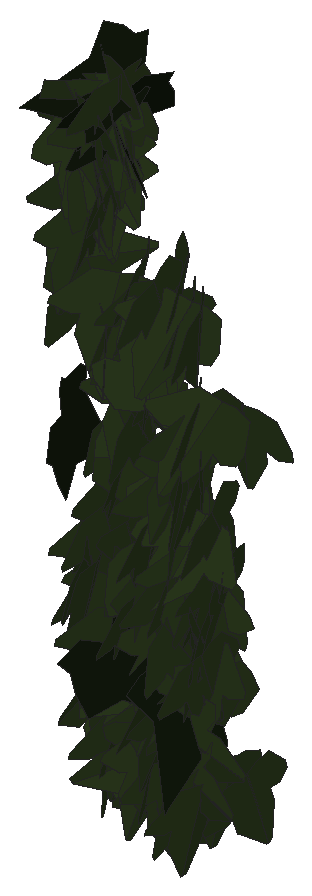
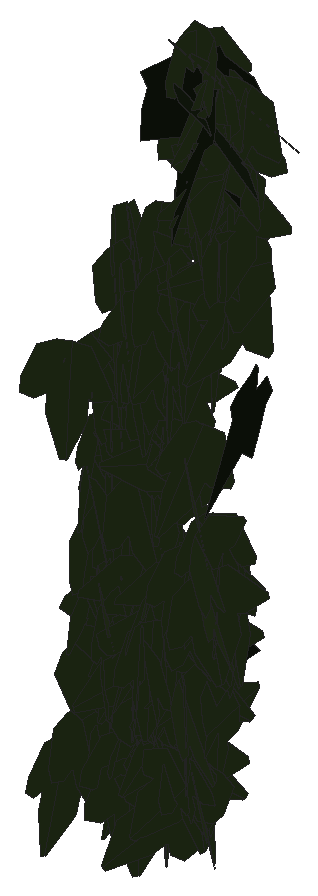
# SketchUp Ruby script. Lengths in inches.
U = 1.inch
M = Sketchup.active_model
def pt(a) = Geom::Point3d.new(a.map { |v| v * U })
def face(e, loops, mat)
  f = e.add_face(loops[0].map { |a| pt(a) })
  loops[1..].each { |l| e.add_face(l.map { |a| pt(a) }).erase! }
  f.material = f.back_material = mat if mat
  f
end
# faces: each face lists its corners as indices into pts; further lists are holes
def faces(e, pts, list, mat = nil) = list.each { |f| face(e, (f[0].is_a?(Array) ? f : [f]).map { |l| l.map { |i| pts[i] } }, mat) }
# xy, xz, yz: faces in a plane at the given z, y or x. An outline is a flat list of corners, or four numbers for a rectangle; further outlines are holes
def ring(l) = l.size == 4 ? [[l[0], l[1]], [l[2], l[1]], [l[2], l[3]], [l[0], l[3]]] : l.each_slice(2).to_a
def flat(e, list, mat, &to3) = list.each { |f| face(e, (f[0].is_a?(Array) ? f : [f]).map { |l| ring(l).map { |u, v| to3.(u, v) } }, mat) }
def xy(e, z, list, mat = nil) = flat(e, list, mat) { |x, y| [x, y, z] }
def xz(e, y, list, mat = nil) = flat(e, list, mat) { |x, z| [x, y, z] }
def yz(e, x, list, mat = nil) = flat(e, list, mat) { |y, z| [x, y, z] }
def lines(e, pts, list) = list.each { |a, b| e.add_line(pt(pts[a]), pt(pts[b])) }
# prism: a flat outline (further loops are holes) pulled along v
def prism(e, loops, v, mat = nil)
  f = face(e, loops, mat); d = Geom::Vector3d.new(v.map { |x| x * U })
  f.pushpull(f.normal.samedirection?(d) ? d.length : -d.length)
end
def box(e, o, s, mat = nil) = prism(e, [[o, [o[0] + s[0], o[1], o[2]], [o[0] + s[0], o[1] + s[1], o[2]], [o[0], o[1] + s[1], o[2]]]], [0, 0, s[2]], mat)
def at(x, y, z, deg = 0) = Geom::Transformation.translation(pt([x, y, z])) * Geom::Transformation.rotation(ORIGIN, Z_AXIS, deg.degrees)
def axes(o, x, y, z) = Geom::Transformation.new([*x, 0, *y, 0, *z, 0, *pt(o).to_a, 1])
def part(name) = M.definitions.add(name)
# library, detail: a bought-in or finely detailed component or shape, given as its bounding box
def library(name, o, s) = part(name).tap { |d| box(d.entities, o, s) }
def detail(e, o, s) = box(e.add_group.entities, o, s)
def put(e, d, t, mat = nil) = e.add_instance(d, t).tap { |i| i.material = mat if mat }
def group(e, t, mat = nil) = e.add_group.tap { |g| g.transformation = t; g.material = mat if mat }.entities
root = M.entities
M.materials.add("efeu1").color = [18, 25, 13]
M.materials.add("efeu2").color = [43, 57, 29]
c1 = part("ivyleaf_10")
p = [[0,0.5,-0.03],[-0.0625,2.02,-0.43],[-0.19,2.01,-0.46],[-0.54,1.05,-0.29],[-0.52,0.625,-0.18],[-0.83,0.76,-0.28],
  [-1.16,0.64,-0.33],[-1.15,0.33,-0.24],[-0.77,-0.39,0.02],[-0.3,-0.51,0.16],[0.04,-0.48,0.23],[-0.02,2.01,-0.4375],
  [-0.06,2.01,-0.43],[0.04,-0.49,0.23],[0.67,-0.49,0.14],[1.38,0.36,-0.2],[1.375,0.51,-0.24],[0.81,0.65,-0.19],
  [0.62,0.59,-0.15],[0.6,1.09,-0.28],[0.5,1.23,-0.31]]
faces(c1.entities,p,[[0,1,2,3,4,5,6,7,8,9,10],[11,12,0,13,14,15,16,17,18,19,20]],"efeu2")
c2 = part("ivyleaf_9")
p = [[1.54,2.16,1.25],[1.36,2.04,1.19],[-0.21,0.99,0.68],[-0.71,1.11,0.82],[-0.85,0.86,0.67],[-0.8,0.17,0.21],
  [-0.9,-0.01,0.1],[-0.67,-0.16,-0.02],[-0.08,-0.08,-0.05],[-0.03,-0.6,-0.4],[0.65,-0.88,-0.66],[0.83,-0.6,-0.49],
  [1.29,-0.42,-0.43],[1.8125,-0.07,-0.26],[1.21,0.44,0.15]]
faces(c2.entities,p,[[0,1,2,3,4,5,6,7,8,9,10,11,12,13,14]],"efeu1")
put(root,c1,axes([11.7,225.35,216.89],[-0.17857,-0.46173,0.07016],[0.01212,-0.07967,-0.49346],[0.46687,-0.17454,0.03964]))
put(root,c1,axes([11.74,225.21,216.97],[0.16413,-0.47089,0.03635],[0.00143,-0.03798,-0.49855],[0.47229,0.16376,-0.01112]))
put(root,c1,axes([11.82,224.86,221.38],[-0.39838,-0.30173,0.01575],[-0.01265,-0.00938,-0.49975],[0.30188,-0.39858,-0.00016]))
put(root,c1,axes([11.73,225.29,217.39],[0.11032,-0.44113,0.20794],[0.06177,-0.19884,-0.45459],[0.48375,0.12599,0.01063]))
put(root,c1,axes([11.78,224.85,220.93],[-0.07095,-0.43919,0.2282],[0.07533,-0.23743,-0.43353],[0.48917,-0.02713,0.09986]))
put(root,c1,axes([11.84,225.46,215.62],[0.11046,-0.48106,0.07989],[0.00859,-0.07998,-0.49349],[0.48757,0.11039,-0.0094]))
put(root,c2,axes([11.9,224.29,218.81],[0.12477,-0.03223,-0.48311],[-0.37094,0.31428,-0.11676],[0.31119,0.38754,0.05452]))
put(root,c1,axes([11.77,224.71,220.16],[-0.14135,-0.32481,-0.35287],[0.14656,0.32103,-0.3542],[0.45667,-0.20356,0.00445]))
put(root,c1,axes([11.9,224.64,216.87],[0.05893,-0.33516,-0.36632],[-0.04723,0.36344,-0.34012],[0.49426,0.07469,0.01118]))
put(root,c1,axes([11.87,224.78,216.61],[0.0968,-0.48951,-0.03181],[-0.00242,0.03195,-0.49897],[0.49054,0.09675,0.00381]))
put(root,c1,axes([11.77,224.7,222.57],[-0.4744,-0.04279,-0.15202],[0.15347,-0.01139,-0.47573],[0.03725,-0.49804,0.02394]))
put(root,c1,axes([11.86,225.47,215.66],[0.23212,-0.41432,-0.15639],[-0.00102,0.17606,-0.46798],[0.44285,0.21758,0.08089]))
put(root,c1,axes([11.8125,225.09,215.1875],[-0.04659,0.03065,-0.49688],[-0.01642,-0.49887,-0.02923],[-0.49755,0.0136,0.04749]))
put(root,c1,axes([11.86,224.875,221.74],[-0.28903,0.40568,-0.04344],[-0.00216,-0.05475,-0.49699],[-0.40799,-0.2871,0.0334]))
put(root,c2,axes([12.22,224.72,222.37],[-0.19027,0.37137,0.27547],[-0.20623,0.19845,-0.40999],[-0.41385,-0.26963,0.07765]))
put(root,c1,axes([11.96,225.22,216.58],[-0.10841,-0.45411,0.17896],[-0.0212,-0.17877,-0.46647],[0.48765,-0.10872,0.01951]))
put(root,c1,axes([11.82,224.77,221.83],[-0.4552,0.11573,-0.17145],[0.1371,-0.14153,-0.45953],[-0.1549,-0.46538,0.09712]))
put(root,c1,axes([11.6875,224.625,220.59],[-0.0317,-0.04118,-0.49729],[0.34536,0.35785,-0.05165],[0.36017,-0.34676,0.00576]))
put(root,c1,axes([11.89,224.71,222.08],[0.47557,0.14781,-0.04451],[-0.06545,0.06248,-0.49175],[-0.13981,0.47355,0.07877]))
put(root,c1,axes([11.86,224.86,221.53],[0.02828,0.49288,0.07916],[-0.00436,0.07953,-0.49362],[-0.49918,0.02723,0.00879]))
put(root,c1,axes([11.89,225.22,214.49],[0.26255,-0.42121,0.06046],[0.06203,-0.03241,-0.49508],[0.42098,0.26746,0.03523]))
put(root,c1,axes([11.99,224.7,221.3],[0.18623,-0.38989,-0.25159],[-0.0422,0.25575,-0.42757],[0.4621,0.18049,0.06235]))
put(root,c1,axes([11.87,224.92,221.62],[0.14253,0.47795,0.0353],[0.0153,0.03228,-0.49872],[-0.47901,0.14324,-0.00543]))
put(root,c2,axes([12.31,224.76,222.93],[-0.41203,0.23888,0.15221],[-0.16527,0.01546,-0.47164],[-0.23004,-0.43897,0.06622]))
put(root,c1,axes([11.99,224.57,222.52],[-0.41687,0.27608,0.00038],[0.00032,0.00117,-0.5],[-0.27608,-0.41687,-0.00115]))
put(root,c1,axes([11.99,224.9,217.32],[-0.06332,-0.46543,-0.17136],[0.07804,0.16125,-0.46681],[0.4898,-0.08586,0.05223]))
put(root,c1,axes([12.05,225.15,214.67],[-0.09041,-0.491,0.02737],[0.01637,-0.03082,-0.49878],[0.49149,-0.0893,0.02165]))
put(root,c1,axes([11.78,224.93,221.86],[0.36756,0.20326,0.27127],[0.21144,0.17526,-0.41782],[-0.26493,0.42187,0.04288]))
put(root,c1,axes([12.06,225.21,217.03],[-0.1396,-0.44702,-0.17517],[0.04992,0.16792,-0.46831],[0.47751,-0.14824,-0.00225]))
put(root,c1,axes([12.14,224.92,216.05],[-0.18571,-0.45465,0.09381],[-0.01438,-0.09535,-0.49061],[0.46401,-0.18492,0.02234]))
put(root,c1,axes([12.03,225.1,218.49],[-0.07518,-0.40489,-0.28357],[0.12073,0.2631,-0.40768],[0.47935,-0.12977,0.05821]))
put(root,c1,axes([12.15,224.63,219.82],[0.27561,-0.2664,-0.32105],[-0.10337,0.32917,-0.36189],[0.40417,0.26585,0.12637]))
put(root,c1,axes([12.11,224.96,221.53],[0.14162,-0.46694,-0.10911],[-0.01395,0.10971,-0.48761],[0.47932,0.14116,0.01805]))
put(root,c1,axes([12.11,225.05,218.07],[0.24396,-0.43277,-0.05648],[-0.01288,0.05754,-0.49651],[0.43625,0.24371,0.01692]))
put(root,c2,axes([12.19,224.82,222.4],[0.28676,0.01346,-0.40937],[-0.39923,0.12087,-0.27569],[0.09154,0.48498,0.08007]))
put(root,c1,axes([11.86,225.34,214.63],[0.26831,0.24909,0.34054],[0.21725,0.26439,-0.36456],[-0.36168,0.34359,0.03364]))
put(root,c1,axes([12.42,224.94,216.54],[-0.32834,0.02811,0.37603],[-0.37511,0.02655,-0.32953],[-0.03849,-0.4985,0.00366]))
put(root,c1,axes([12.17,224.79,222.375],[-0.27662,-0.41372,0.04816],[0.02211,-0.07232,-0.49425],[0.41592,-0.27131,0.0583]))
put(root,c1,axes([12.17,225,219.88],[0.06136,-0.46995,-0.15931],[0.0263,0.16338,-0.47182],[0.49552,0.04952,0.04477]))
put(root,c2,axes([12.31,224.77,222.75],[-0.01911,0.42881,-0.25644],[-0.0113,-0.25693,-0.42879],[-0.49951,-0.01059,0.01951]))
put(root,c1,axes([12.33,225.1,215.57],[0.25511,0.18186,-0.38967],[-0.31292,-0.23227,-0.31326],[-0.29496,0.40371,-0.0047]))
put(root,c1,axes([12.12,224.8,222.38],[-0.11924,0.48341,-0.04581],[0.00443,-0.04608,-0.49785],[-0.48555,-0.11913,0.00671]))
put(root,c1,axes([12.23,225.22,215.54],[-0.15709,-0.45485,0.13578],[0.01622,-0.14808,-0.47729],[0.4744,-0.14556,0.06128]))
put(root,c1,axes([12.23,224.77,220.27],[-0.31528,-0.36096,0.1425],[0.01916,-0.19785,-0.45879],[0.3876,-0.28384,0.13858]))
put(root,c1,axes([12.11,225.44,214.81],[0.48585,-0.11243,0.03617],[0.03624,-0.00384,-0.49867],[0.11241,0.48718,0.00442]))
put(root,c1,axes([12.1,224.73,222.6875],[-0.44305,0.10276,-0.20772],[0.142,-0.2338,-0.41854],[-0.18315,-0.42986,0.17798]))
put(root,c1,axes([12.24,224.79,222.56],[-0.24143,0.43682,0.02996],[-0.02765,0.01894,-0.49888],[-0.43698,-0.24254,0.01502]))
put(root,c1,axes([12.24,224.72,223.02],[-0.39495,0.29622,-0.07919],[0.04186,-0.07584,-0.49244],[-0.30375,-0.3956,0.0351]))
put(root,c1,axes([12.18,225.25,215.24],[-0.11074,-0.35966,-0.32921],[0.19214,0.27809,-0.36844],[0.44813,-0.20812,0.07662]))
put(root,c1,axes([12.3,225.1,220.42],[0.19276,-0.45725,-0.0614],[-0.00466,0.06461,-0.49579],[0.46133,0.1917,0.02065]))
put(root,c1,axes([12.31,225.48,216.15],[-0.12834,-0.47237,-0.10196],[0.03531,0.09604,-0.48942],[0.48196,-0.13283,0.00871]))
put(root,c1,axes([12.61,225.01,214.54],[0.20201,0.11662,-0.44226],[-0.43612,-0.09656,-0.22467],[-0.13782,0.47652,0.06271]))
put(root,c1,axes([12.1,225.36,214.17],[0.23558,0.20855,0.3886],[0.21214,0.33266,-0.30714],[-0.38665,0.30958,0.06825]))
put(root,c1,axes([12.46,225.05,219.03],[-0.33195,-0.31877,0.19544],[-0.06624,-0.20708,-0.45026],[0.368,-0.32482,0.09524]))
put(root,c1,axes([12.39,224.59,222.93],[-0.07749,-0.48516,-0.09283],[0.02034,0.09075,-0.49127],[0.49354,-0.07991,0.00567]))
put(root,c1,axes([12.43,224.8125,216.42],[0.09581,-0.47999,-0.10213],[-0.01398,0.10135,-0.48942],[0.49053,0.09664,0.006]))
put(root,c1,axes([12.35,225.55,216.02],[0.40714,-0.29006,0.01],[0.05538,0.06073,-0.4932],[0.2849,0.40271,0.08158]))
put(root,c1,axes([12.5,225.07,215.21],[0.08449,-0.4612,-0.17366],[-0.05038,0.16719,-0.46852],[0.49023,0.09667,-0.01822]))
put(root,c1,axes([12.5,225.07,220.21],[-0.09235,-0.48704,0.06531],[-0.00074,-0.06632,-0.49558],[0.4914,-0.09163,0.01153]))
put(root,c1,axes([12.36,225.04,216.8],[0.13746,0.47717,0.05843],[0.01659,0.05603,-0.49657],[-0.48045,0.13846,-0.00043]))
put(root,c1,axes([12.49,225.09,214.41],[0.24604,-0.39771,-0.17688],[-0.03368,0.18518,-0.46322],[0.43397,0.23986,0.06433]))
put(root,c1,axes([12.6875,225.33,215.45],[-0.20477,-0.19889,0.4105],[-0.22418,-0.348,-0.28043],[0.39726,-0.2989,0.05334]))
put(root,c1,axes([12.47,225.21,214.46],[-0.11519,-0.42075,0.24434],[0.07751,-0.26376,-0.41764],[0.48034,-0.05834,0.12598]))
put(root,c1,axes([12.5,225.48,216.1],[0.26301,-0.35921,-0.22758],[-0.02287,0.25526,-0.42932],[0.42462,0.23624,0.11784]))
put(root,c1,axes([12.53,225.01,219.46],[-0.1429,-0.46934,0.09646],[0.02579,-0.10804,-0.48751],[0.47845,-0.13435,0.05509]))
put(root,c1,axes([12.18,224.9,218.18],[-0.04808,-0.01631,-0.49742],[0.44719,0.21791,-0.05037],[0.21843,-0.44972,-0.00637]))
put(root,c1,axes([12.55,224.9,219.4],[0.2943,-0.34399,-0.21228],[-0.03936,0.23694,-0.43853],[0.40229,0.27482,0.11239]))
put(root,c2,axes([12.3125,224.63,215.95],[-0.03133,-0.11281,-0.4861],[0.16898,0.45588,-0.11669],[0.46953,-0.1716,0.00956]))
put(root,c1,axes([12.55,225.3,216.3],[0.11156,-0.40822,-0.2663],[0.0924,0.28594,-0.39962],[0.47856,0.03995,0.13924]))
put(root,c1,axes([12.66,225.26,217.74],[-0.17964,-0.4569,0.09471],[-0.0148,-0.09585,-0.4905],[0.46638,-0.17903,0.02091]))
put(root,c1,axes([12.62,224.59,218.9],[0.06869,-0.38267,-0.3144],[0.01754,0.31909,-0.38454],[0.49495,0.04179,0.05726]))
put(root,c1,axes([12.46,225.26,215.8],[0.10388,0.0892,0.48089],[0.08852,0.48007,-0.10817],[-0.48101,0.10761,0.08394]))
put(root,c1,axes([12.61,225.15,219.93],[-0.23462,-0.39609,-0.1951],[0.08756,0.17481,-0.46019],[0.43276,-0.25011,-0.01267]))
put(root,c1,axes([12.6,225.25,216.04],[0.04804,0.39124,0.30761],[-0.02582,0.31058,-0.39099],[-0.49702,0.02168,0.05005]))
put(root,c1,axes([12.71,224.78,217.5],[0.11997,-0.47747,-0.08734],[-0.00617,0.08846,-0.49207],[0.48536,0.11914,0.01533]))
put(root,c1,axes([12.8125,225.11,216.01],[-0.23104,-0.38865,0.21348],[-0.07507,-0.20296,-0.45075],[0.43702,-0.24033,0.03543]))
put(root,c1,axes([12.43,224.79,219.64],[0.37974,0.12884,0.29867],[0.27433,0.11982,-0.40048],[-0.17477,0.46802,0.02031]))
put(root,c1,axes([12.76,225.11,219.32],[0.04343,-0.48297,-0.12186],[-0.01123,0.12135,-0.48492],[0.49798,0.04486,-0.00031]))
put(root,c1,axes([12.75,224.64,219.37],[0.18629,0.46399,-0.00285],[0.00103,0.00265,0.49999],[0.464,-0.1863,0.00003]))
put(root,c1,axes([12.82,225.11,214.14],[-0.36164,-0.34518,0.00857],[-0.00542,-0.00673,-0.49993],[0.34524,-0.36167,0.00113]))
put(root,c1,axes([12.67,225.26,216.84],[0.15426,0.46817,0.08381],[0.00074,0.08788,-0.49222],[-0.47561,0.15198,0.02642]))
put(root,c1,axes([12.79,224.94,216.73],[-0.32618,-0.37176,-0.07348],[0.05142,0.05263,-0.49456],[0.37545,-0.33018,0.0039]))
put(root,c1,axes([12.69,225.08,216.41],[-0.12521,-0.32839,-0.35565],[0.1867,0.30617,-0.34843],[0.44662,-0.22005,0.04595]))
put(root,c1,axes([12.86,225.46,216.23],[0.03439,-0.46726,-0.17459],[0.00122,0.17509,-0.46834],[0.49881,0.03178,0.01318]))
put(root,c1,axes([12.5625,225.16,218.15],[0.38723,0.12393,0.29103],[0.25496,0.15,-0.40311],[-0.18723,0.46059,0.05297]))
put(root,c1,axes([12.72,225.16,214.7],[0.27436,-0.31209,0.27807],[0.20825,-0.18634,-0.41462],[0.36243,0.34333,0.02774]))
put(root,c1,axes([13.21,225.47,215.65],[-0.25754,-0.07725,0.42155],[-0.37396,-0.19973,-0.26507],[0.20935,-0.45182,0.0451]))
put(root,c1,axes([12.92,224.89,215.27],[0.06105,-0.47705,0.13673],[0.00065,-0.13769,-0.48067],[0.49626,0.05887,-0.0162]))
put(root,c1,axes([12.9,224.99,216.68],[-0.39379,0.30799,0.00859],[-0.00486,0.00772,-0.49992],[-0.30807,-0.39381,-0.00309]))
put(root,c1,axes([12.93,225.04,214.42],[-0.30919,-0.38377,-0.08438],[0.05719,0.06228,-0.4928],[0.38875,-0.31439,0.00538]))
put(root,c1,axes([12.95,225.12,220.125],[0.19475,-0.45122,-0.09205],[0.00887,0.1036,-0.48907],[0.46043,0.18886,0.04836]))
put(root,c1,axes([12.95,224.55,220.62],[-0.01572,-0.44709,-0.22331],[0.04534,0.22122,-0.4461],[0.49769,-0.03427,0.03359]))
put(root,c1,axes([13.01,225.39,216.55],[0.20504,-0.44577,-0.09619],[-0.04263,0.08627,-0.49065],[0.45403,0.2094,-0.00263]))
put(root,c1,axes([13,224.95,220.75],[0.25821,-0.40021,-0.1522],[-0.03706,0.15618,-0.47353],[0.42656,0.25582,0.05099]))
put(root,c1,axes([12.9,225.36,216.38],[-0.47488,-0.06954,-0.14018],[0.1522,-0.1012,-0.4654],[0.03635,-0.48469,0.11728]))
put(root,c1,axes([13.01,224.89,216.9375],[0.10308,-0.45738,-0.17372],[0.00338,0.17819,-0.46716],[0.48925,0.09513,0.03983]))
put(root,c1,axes([13.14,224.79,220.25],[-0.33323,-0.2728,0.25404],[-0.08132,-0.27934,-0.40664],[0.36379,-0.31233,0.1418]))
put(root,c1,axes([13.05,225.1,215.9],[0.23674,-0.37435,-0.23198],[-0.0029,0.26205,-0.42582],[0.44039,0.20296,0.12191]))
put(root,c1,axes([13.11,224.95,218.45],[-0.07865,-0.41668,0.26493],[0.03957,-0.27273,-0.4172],[0.49219,-0.04465,0.07588]))
put(root,c1,axes([13.05,224.6875,216.35],[0.04961,-0.40421,-0.29009],[0.11297,0.29307,-0.38903],[0.48454,-0.02694,0.12041]))
put(root,c1,axes([13.13,224.71,216.91],[-0.2141,-0.43776,-0.11193],[0.03741,0.10627,-0.48714],[0.45029,-0.21697,-0.01275]))
put(root,c1,axes([13.28,225.04,215.54],[-0.15612,-0.29742,0.37036],[-0.15294,-0.33761,-0.3356],[0.44971,-0.21807,0.01444]))
put(root,c1,axes([13.14,224.77,214.32],[0.0437,-0.41534,-0.27492],[0.07771,0.27828,-0.40807],[0.49199,-0.00706,0.08888]))
put(root,c1,axes([13.21,224.92,218.78],[-0.05356,-0.4646,0.17687],[0.00656,-0.17854,-0.46699],[0.49708,-0.0477,0.02522]))
put(root,c1,axes([13.26,224.55,218.38],[0.21495,-0.31404,-0.32431],[-0.08792,0.32319,-0.37124],[0.4428,0.21662,0.08372]))
put(root,c2,axes([13.05,225,215.43],[-0.02338,-0.47419,0.15684],[-0.01056,-0.15651,-0.47476],[0.49934,-0.02552,-0.0027]))
put(root,c1,axes([13.26,224.91,217.17],[-0.1694,-0.44472,0.15338],[0.00833,-0.16583,-0.47162],[0.47036,-0.15723,0.06359]))
put(root,c1,axes([13.25,224.85,219.06],[0.17785,-0.43292,-0.17592],[-0.0286,0.17779,-0.46645],[0.46642,0.17598,0.03848]))
put(root,c1,axes([13.05,224.92,218.02],[0.20632,-0.30168,0.3412],[0.23416,-0.25102,-0.36354],[0.39064,0.3098,0.0377]))
put(root,c1,axes([13.3,224.77,217.64],[0.45071,0.10303,-0.19037],[-0.18331,-0.05218,-0.46225],[-0.11512,0.48648,-0.00926]))
put(root,c1,axes([13.27,225.04,216.41],[0.20764,-0.41617,-0.18355],[-0.00611,0.1992,-0.45857],[0.4548,0.19268,0.07764]))
put(root,c1,axes([13.34,224.78,218.25],[0.13561,-0.38687,-0.28625],[-0.0597,0.28158,-0.40884],[0.47754,0.14506,0.03018]))
put(root,c1,axes([13.33,225.25,216.95],[0.02481,-0.49937,-0.00388],[-0.0022,0.00377,-0.49998],[0.49938,0.02482,-0.00201]))
put(root,c1,axes([13.3,225.19,217.47],[0.37445,-0.31863,-0.09087],[-0.03518,0.09812,-0.48902],[0.32946,0.37262,0.05106]))
put(root,c1,axes([13.23,225.48,216.5],[-0.04418,0.29484,-0.4014],[0.00759,-0.40253,-0.2965],[-0.49799,-0.03229,0.03109]))
put(root,c1,axes([13.45,224.9,219.07],[-0.31462,-0.26426,0.28492],[-0.0984,-0.30047,-0.38734],[0.37594,-0.29981,0.13706]))
put(root,c1,axes([13.22,225.0625,215.91],[0.49206,-0.0398,0.0793],[0.07856,-0.01225,-0.49364],[0.04123,0.49826,-0.0058]))
put(root,c1,axes([13.39,224.75,214.37],[-0.04985,-0.49653,0.03124],[0.0044,-0.03183,-0.49897],[0.49749,-0.04947,0.00754]))
put(root,c1,axes([13.43,224.79,216.03],[-0.08197,-0.45124,-0.19915],[0.04995,0.19325,-0.45843],[0.4907,-0.09505,0.0134]))
put(root,c1,axes([13.48,225.17,214.57],[-0.14419,-0.4756,0.05491],[-0.00759,-0.05506,-0.4969],[0.4787,-0.14413,0.00866]))
put(root,c1,axes([13.11,224.87,214.6],[-0.07142,0.0321,-0.49383],[0.40953,-0.27627,-0.07719],[-0.27782,-0.4155,0.01317]))
put(root,c1,axes([13.49,224.59,220.4],[0.17067,-0.44584,-0.14866],[0.00312,0.15923,-0.47396],[0.46996,0.16085,0.05714]))
put(root,c1,axes([13.11,224.91,215.02],[-0.05911,0.04153,-0.49475],[0.44254,-0.22148,-0.07146],[-0.22509,-0.44634,-0.01057]))
put(root,c1,axes([13.54,225.45,214.3],[-0.09237,-0.45298,-0.19046],[0.06626,0.18054,-0.46153],[0.48691,-0.1105,0.02667]))
put(root,c1,axes([13.58,224.78,217.92],[0.01475,-0.4092,-0.28694],[0.01217,0.28727,-0.40906],[0.49963,0.00508,0.01843]))
put(root,c1,axes([13.67,225.26,218.99],[-0.4905,0.01185,0.09626],[-0.09631,-0.00091,-0.49064],[-0.01145,-0.49986,0.00317]))
